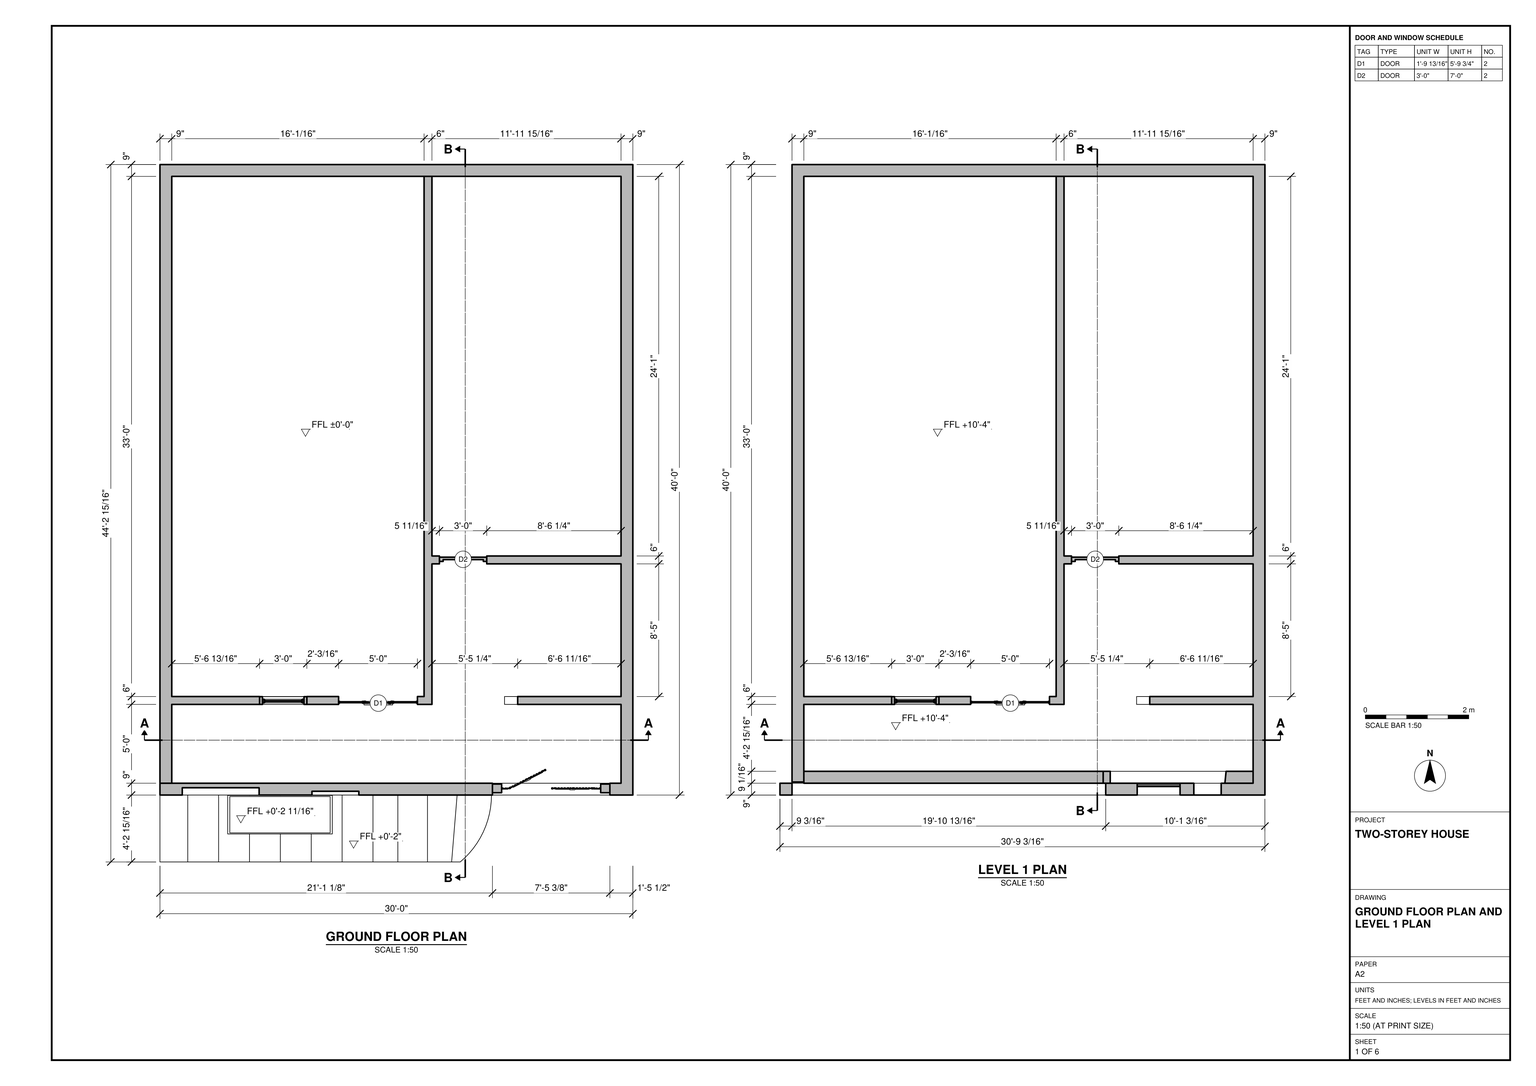
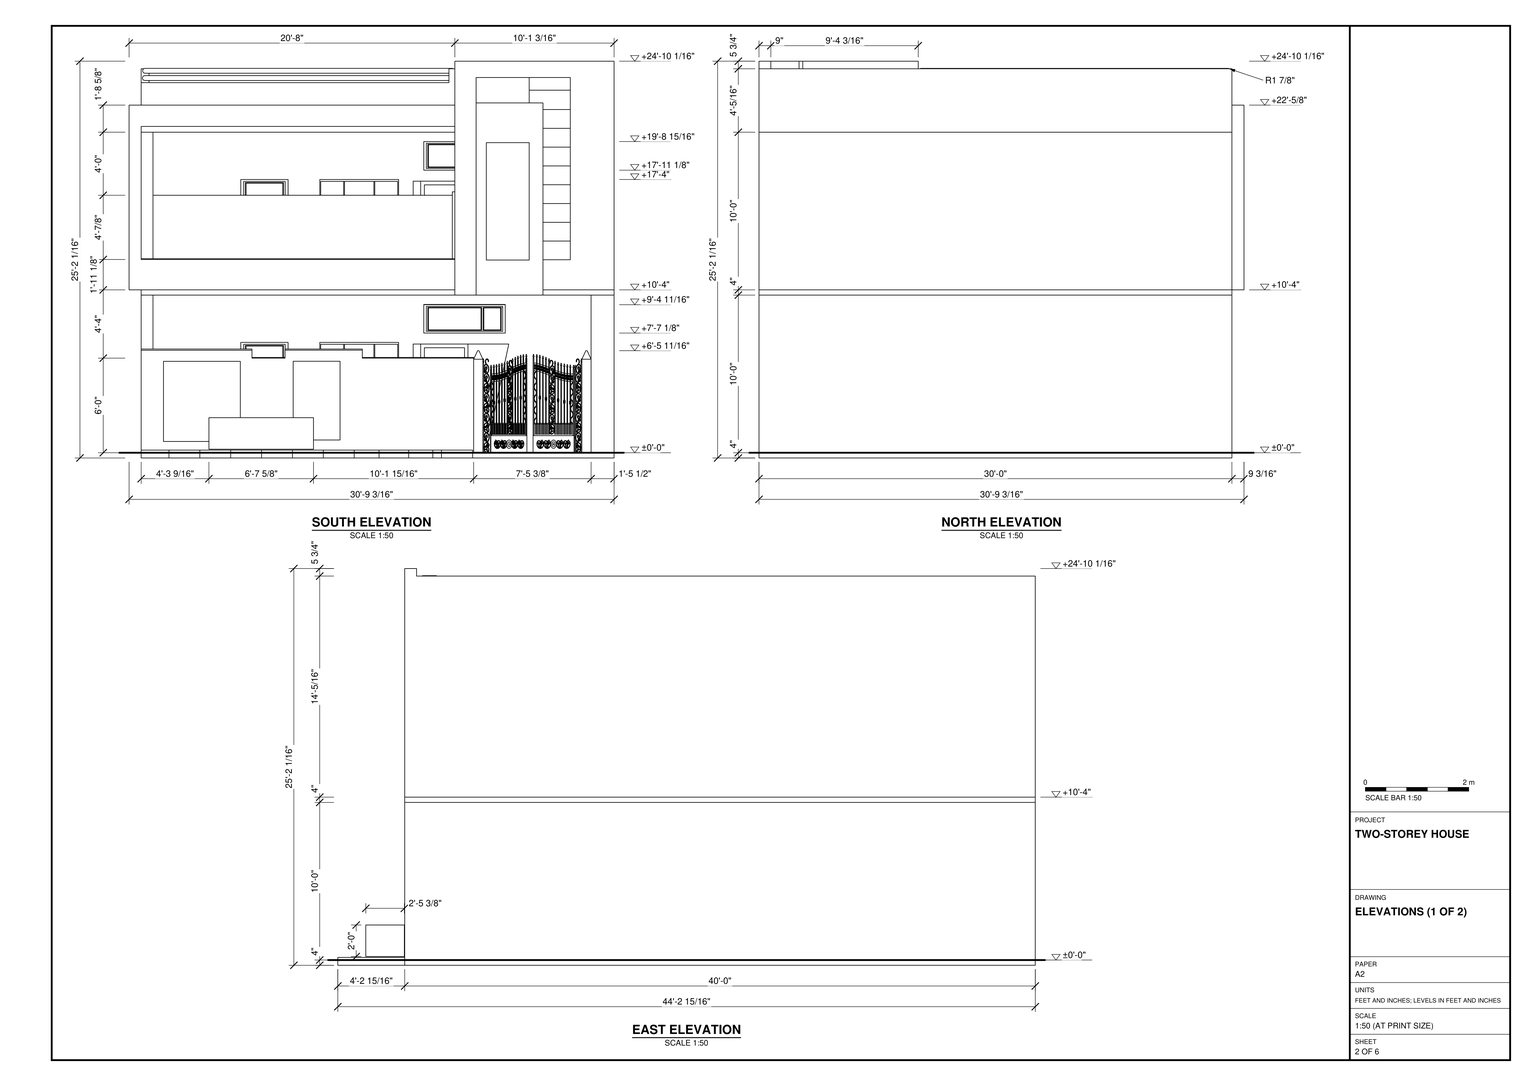
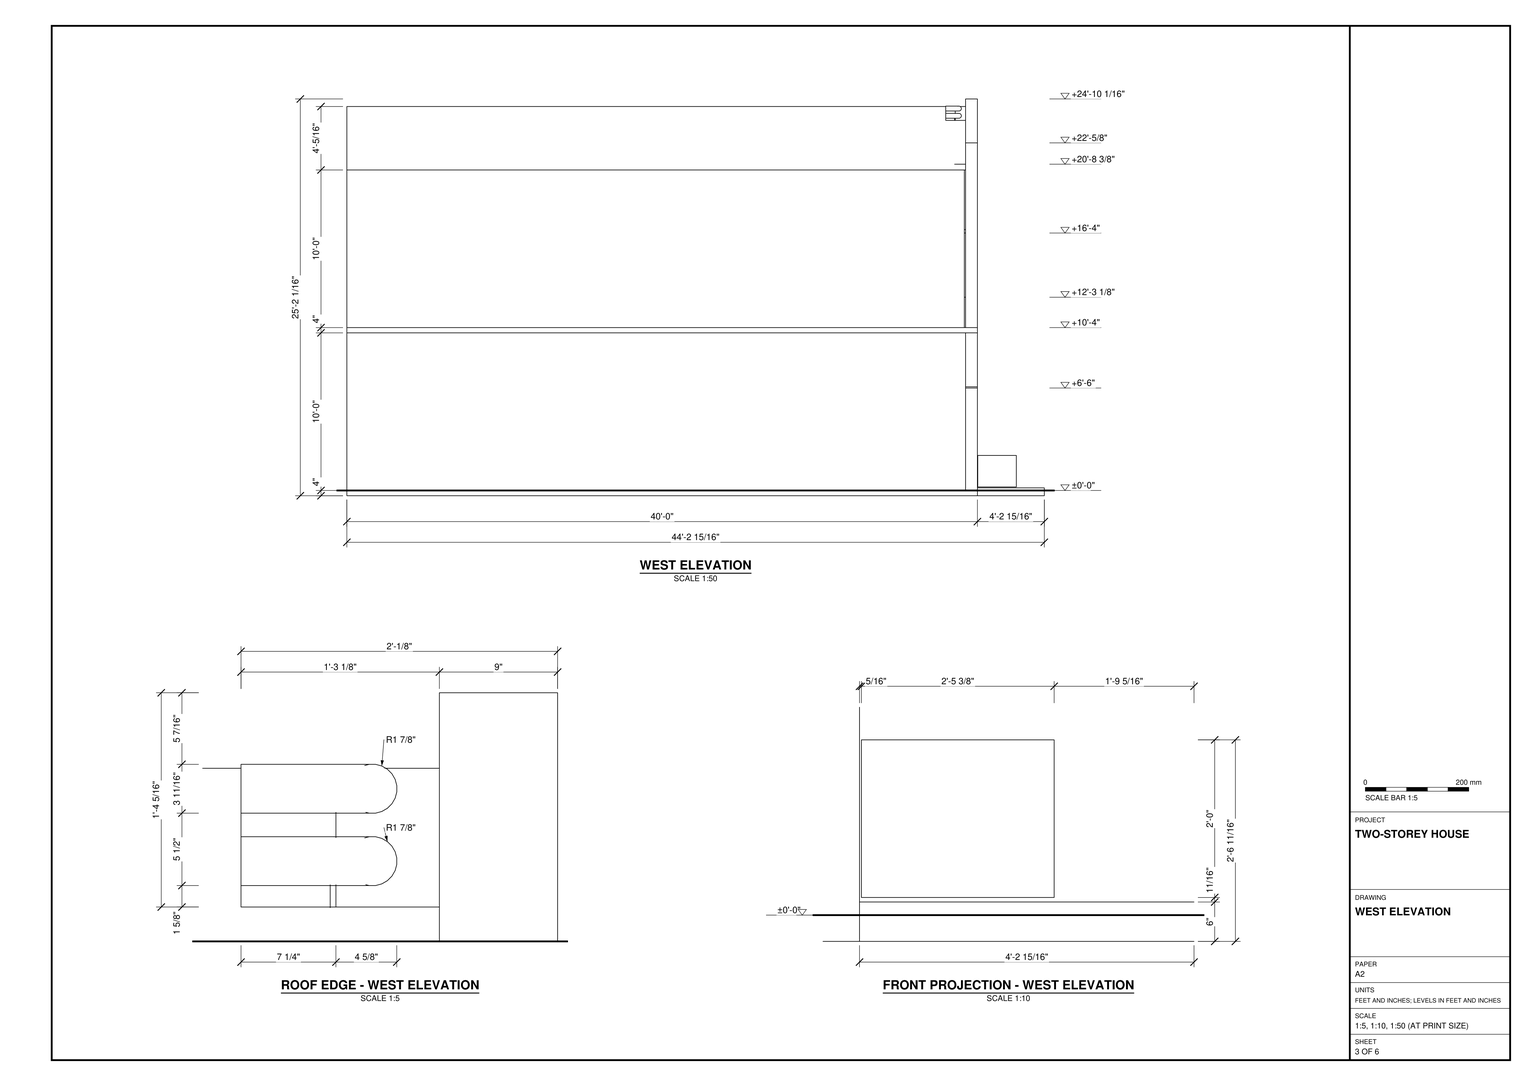
Build the two-storey house in SketchUp using task_files/diagram_01.pdf. Work in feet and inches. Orient the entrance to the south. The overall model, including the front projection and roof edge, measures 30'-9 3/16" east to west, 44'-2 15/16" north to south and 25'-2 1/16" high. Set the ground finished floor at ±0'-0" and the upper finished floor at +10'-4".

Lay out the 9" exterior walls and 6" internal partitions from the plans. On each floor, keep the large room to the west and divide the narrower eastern bay with a cross wall. Model the floor slabs, doors and windows, using the plans to locate the openings and the elevations to set their heights.

At the south entrance, model the projecting paved strip, low solid front wall and paired gate. Above them, form the recessed balcony with its solid front, surrounding rectangular frame and taller panel over the gate. Follow the roof-edge detail for the horizontal bands and their rounded profile.

Keep walls, slabs, roof and each furniture or joinery piece shown in separate groups or components, and use components for repeated parts. Decor and loose items, where shown, may be any suitable library components. Save one SketchUp model as output_files/two_storey_house_with_a_gated_entrance_and_balcony.skp.

# SketchUp Ruby script. Lengths in inches.
U = 1.inch
M = Sketchup.active_model
def pt(a) = Geom::Point3d.new(a.map { |v| v * U })
def face(e, loops, mat)
  f = e.add_face(loops[0].map { |a| pt(a) })
  loops[1..].each { |l| e.add_face(l.map { |a| pt(a) }).erase! }
  f.material = f.back_material = mat if mat
  f
end
# faces: each face lists its corners as indices into pts; further lists are holes
def faces(e, pts, list, mat = nil) = list.each { |f| face(e, (f[0].is_a?(Array) ? f : [f]).map { |l| l.map { |i| pts[i] } }, mat) }
# xy, xz, yz: faces in a plane at the given z, y or x. An outline is a flat list of corners, or four numbers for a rectangle; further outlines are holes
def ring(l) = l.size == 4 ? [[l[0], l[1]], [l[2], l[1]], [l[2], l[3]], [l[0], l[3]]] : l.each_slice(2).to_a
def flat(e, list, mat, &to3) = list.each { |f| face(e, (f[0].is_a?(Array) ? f : [f]).map { |l| ring(l).map { |u, v| to3.(u, v) } }, mat) }
def xy(e, z, list, mat = nil) = flat(e, list, mat) { |x, y| [x, y, z] }
def xz(e, y, list, mat = nil) = flat(e, list, mat) { |x, z| [x, y, z] }
def yz(e, x, list, mat = nil) = flat(e, list, mat) { |y, z| [x, y, z] }
def lines(e, pts, list) = list.each { |a, b| e.add_line(pt(pts[a]), pt(pts[b])) }
# prism: a flat outline (further loops are holes) pulled along v
def prism(e, loops, v, mat = nil)
  f = face(e, loops, mat); d = Geom::Vector3d.new(v.map { |x| x * U })
  f.pushpull(f.normal.samedirection?(d) ? d.length : -d.length)
end
def box(e, o, s, mat = nil) = prism(e, [[o, [o[0] + s[0], o[1], o[2]], [o[0] + s[0], o[1] + s[1], o[2]], [o[0], o[1] + s[1], o[2]]]], [0, 0, s[2]], mat)
def at(x, y, z, deg = 0) = Geom::Transformation.translation(pt([x, y, z])) * Geom::Transformation.rotation(ORIGIN, Z_AXIS, deg.degrees)
def axes(o, x, y, z) = Geom::Transformation.new([*x, 0, *y, 0, *z, 0, *pt(o).to_a, 1])
def part(name) = M.definitions.add(name)
# library, detail: a bought-in or finely detailed component or shape, given as its bounding box
def library(name, o, s) = part(name).tap { |d| box(d.entities, o, s) }
def detail(e, o, s) = box(e.add_group.entities, o, s)
def put(e, d, t, mat = nil) = e.add_instance(d, t).tap { |i| i.material = mat if mat }
def group(e, t, mat = nil) = e.add_group.tap { |g| g.transformation = t; g.material = mat if mat }.entities
root = M.entities
M.materials.add("Portão1").color = [45, 31, 24]
M.materials.add("[Color A01]").color = [255, 204, 204]
M.materials.add("[Color C07]").color = [130, 64, 0]
M.materials.add("[Color D07]").color = [153, 114, 0]
M.materials.add("[Color H01]").color = [204, 255, 255]
M.materials.add("[Color H07]").color = [0, 153, 153]
M.materials.add("[Color M00]").color = [255, 255, 255]
M.materials.add("[Color M05]").color = [114, 114, 114]
M.materials.add("[Color M06]").color = [86, 86, 86]
M.materials.add("[Color M08]").color = [30, 30, 30]
M.materials.add("[Diamond Box]").color = [152, 152, 152]
M.materials.add("[Formica Graystone]").color = [149, 146, 135]
M.materials.add("[Formica Speckled Grey]").color = [94, 105, 111]
M.materials.add("[Metal Corrugated Shiny]").color = [193, 193, 193]
M.materials.add("[Metal Embossed]").color = [144, 144, 144]
M.materials.add("[Metal Seamed]").color = [118, 119, 115]
M.materials.add("[Translucent Glass Blue]").color = [100, 149, 237]
M.materials["[Translucent Glass Blue]"].alpha = 0.5
c1 = library("Framed window",[0,0,0],[45.28,5.91,88.58])
c2 = part("puerta")
xy(c2.entities,0,[[122.07,0.28,122.07,2.03,141.26,2.03,141.26,0.28,139.87,0.28,139.87,1.03,123.57,1.03,123.57,0.28]])
xy(c2.entities,34.05,[[123.57,0.28,139.87,1.03]])
xy(c2.entities,35.79,[[122.07,0.28,141.26,2.03]])
xz(c2.entities,0.28,[[122.07,0,123.57,0,123.57,34.05,139.87,34.05,139.87,0,141.26,0,141.26,35.79,122.07,35.79]])
xz(c2.entities,1.03,[[123.57,0,139.87,34.05]])
xz(c2.entities,2.03,[[122.07,0,141.26,35.79]])
yz(c2.entities,122.07,[[0.28,0,2.03,35.79]])
yz(c2.entities,123.57,[[0.28,0,1.03,34.05]])
yz(c2.entities,139.87,[[0.28,0,1.03,34.05]])
yz(c2.entities,141.26,[[0.28,0,2.03,35.79]])
c3 = part("puerta medieval")
put(c3.entities,c2,axes([-167.24,-2.78,0],[2.37,0,0],[0,2.37,0],[0,0,2.37]))
c4 = library("Group\#4",[0,0,0],[50.79,2.36,34.25])
c5 = library("Group\#50",[0,0,0],[18.9,34.65,18.9])
c6 = library("Group\#125",[0,0,0],[24.7,44.27,7.48])
c7 = part("Group\#121")
xy(c7.entities,0,[[0,0,3.91,91.27]])
xy(c7.entities,3.9375,[[0,0,3.91,91.27]])
yz(c7.entities,0,[[0,0,91.27,3.9375]])
yz(c7.entities,3.91,[[0,0,91.27,3.9375]])
c8 = library("Group\#127",[0,0,0],[67.6,135.77,7.48])
c9 = library("Group\#123",[-2.125,-9.89,0],[28.4375,40.22,7.48])
c10 = library("Group\#134",[0.71,0,0],[33.82,463.5,7.48])
c11 = library("Group\#128",[0,0,0],[67.6,87.29,7.48])
c12 = library("Group\#126",[0,0,0],[79.08,92.15,7.48])
c13 = library("Group\#63",[0,0,0],[9.61,9.61,1.97])
c14 = part("Group\#139")
xy(c14.entities,0,[[0,0,15.75,15.75]])
xy(c14.entities,107.61,[[0,0,15.75,15.75]])
xy(c14.entities,117.46,[[6.69,6.69,9.06,9.06]])
xz(c14.entities,0,[[0,0,15.75,107.61]])
xz(c14.entities,15.75,[[0,0,15.75,107.61]])
yz(c14.entities,0,[[0,0,15.75,107.61]])
yz(c14.entities,15.75,[[0,0,15.75,107.61]])
p = [[15.75,0,107.61],[9.06,6.69,117.46],[6.69,6.69,117.46],[0,0,107.61],[6.69,9.06,117.46],[0,15.75,107.61],
  [15.75,15.75,107.61],[9.06,9.06,117.46]]
faces(c14.entities,p,[[0,1,2,3],[2,4,5,3],[1,0,6,7],[5,4,7,6]])
c15 = library("Group\#133",[0,65.85,0],[33.82,371.91,7.48])
c16 = library("Group\#103",[0,-22.71,0],[10.28,108.02,0.97])
c17 = part("Group\#135")
box(c17.entities,[0,-207.47,0],[11.8125,797.23,11.8125])
c18 = library("Group\#130",[0,0,0],[71.84,113.4,4.25])
c19 = part("Group\#146")
xy(c19.entities,0,[[1.62,1.62,1.62,11.86,2.11,11.86,2.11,2.11],[1.62,1.62,2.11,2.11,235.86,2.11,235.86,1.62]],"[Formica Speckled Grey]")
xy(c19.entities,3.72,[[1.61,1.61,2.1,2.1,2.1,11.86,1.61,11.86],[1.61,1.61,235.86,1.61,235.86,2.1,2.1,2.1]],"[Formica Speckled Grey]")
xz(c19.entities,0,[[0,1.61,235.86,2.1]],"[Formica Speckled Grey]")
xz(c19.entities,3.72,[[3.72,1.62,235.86,2.11]],"[Formica Speckled Grey]")
xz(c19.entities,11.86,[[1.62,0,1.14,0.125,0.72,0.37,0.37,0.72,0.13,1.14,0,1.61,0,2.1,0.125,2.58,0.37,3,0.72,3.35,1.14,3.59,1.61,3.72,2.1,3.72,2.58,3.59,3,3.35,3.35,3,3.59,2.58,3.72,2.11,3.72,1.62,3.59,1.14,3.35,0.72,3,0.37,2.58,0.13,2.11,0]],"[Formica Speckled Grey]")
yz(c19.entities,0,[[0,1.61,11.86,2.1]],"[Formica Speckled Grey]")
yz(c19.entities,3.72,[[3.72,1.62,11.86,2.11]],"[Formica Speckled Grey]")
yz(c19.entities,235.86,[[1.62,0,2.11,0,2.58,0.13,3,0.37,3.35,0.72,3.59,1.14,3.72,1.62,3.72,2.11,3.59,2.58,3.35,3,3,3.35,2.58,3.59,2.1,3.72,1.61,3.72,1.14,3.59,0.72,3.35,0.37,3,0.125,2.58,0,2.1,0,1.61,0.13,1.14,0.37,0.72,0.72,0.37,1.14,0.125]],"[Formica Speckled Grey]")
p = [[1.14,11.86,0.125],[1.62,11.86,0],[1.62,1.62,0],[1.14,1.14,0.125],[235.86,1.62,0],[235.86,1.14,0.125],
  [2.11,11.86,0],[2.58,11.86,0.13],[2.58,2.58,0.13],[2.11,2.11,0],[235.86,2.58,0.13],[235.86,2.11,0],
  [0.72,11.86,0.37],[0.72,0.72,0.37],[235.86,0.72,0.37],[3,11.86,0.37],[3,3,0.37],[235.86,3,0.37],
  [0.37,11.86,0.72],[0.37,0.37,0.72],[235.86,0.37,0.72],[3.35,11.86,0.72],[3.35,3.35,0.72],[235.86,3.35,0.72],
  [0.13,11.86,1.14],[0.13,0.13,1.14],[235.86,0.13,1.14],[3.59,11.86,1.14],[3.59,3.59,1.14],[235.86,3.59,1.14],
  [0,11.86,1.61],[0,0,1.61],[235.86,0,1.61],[3.72,11.86,1.62],[3.72,3.72,1.62],[235.86,3.72,1.62],
  [0.125,11.86,2.58],[0,11.86,2.1],[0,0,2.1],[0.125,0.125,2.58],[235.86,0,2.1],[235.86,0.125,2.58],
  [3.72,11.86,2.11],[3.59,11.86,2.58],[3.59,3.59,2.58],[3.72,3.72,2.11],[235.86,3.59,2.58],[235.86,3.72,2.11],
  [0.37,11.86,3],[0.37,0.37,3],[235.86,0.37,3],[3.35,11.86,3],[3.35,3.35,3],[235.86,3.35,3],
  [0.72,11.86,3.35],[0.72,0.72,3.35],[235.86,0.72,3.35],[3,11.86,3.35],[3,3,3.35],[235.86,3,3.35],
  [1.14,11.86,3.59],[1.14,1.14,3.59],[235.86,1.14,3.59],[2.58,11.86,3.59],[2.58,2.58,3.59],[235.86,2.58,3.59],
  [1.61,11.86,3.72],[1.61,1.61,3.72],[235.86,1.61,3.72],[2.1,11.86,3.72],[2.1,2.1,3.72],[235.86,2.1,3.72]]
faces(c19.entities,p,[[0,1,2,3],[3,2,4,5],[6,7,8,9],[9,8,10,11],[12,0,3,13],[13,3,5,14],[7,15,16,8],[8,16,17,10],
  [18,12,13,19],[19,13,14,20],[15,21,22,16],[16,22,23,17],[24,18,19,25],[25,19,20,26],[21,27,28,22],[22,28,29,23],
  [30,24,25,31],[31,25,26,32],[27,33,34,28],[28,34,35,29],[36,37,38,39],[39,38,40,41],[42,43,44,45],[45,44,46,47],
  [48,36,39,49],[49,39,41,50],[43,51,52,44],[44,52,53,46],[54,48,49,55],[55,49,50,56],[51,57,58,52],[52,58,59,53],
  [60,54,55,61],[61,55,56,62],[57,63,64,58],[58,64,65,59],[66,60,61,67],[67,61,62,68],[63,69,70,64],[64,70,71,65]],"[Formica Speckled Grey]")
xy(root,-4,[[9.1875,0,9.1875,50.9375,261.5625,50.9375,261.38,46.11,260.85,41.3,259.97,36.54,258.75,31.87,257.19,27.29,255.31,22.84,253.1,18.53,250.59,14.4,247.79,10.46,244.71,6.73,241.36,3.24,237.77,0],[9.1875,50.9375,369.1875,530.9375]])
xy(root,0,[[351.7,50.9375,351.7,59.9375,360.1875,59.9375,360.1875,119.9375,271.49,119.9375,271.49,125.9375,360.1875,125.9375,360.1875,226.9375,257.96,226.9375,257.96,232.9375,360.1875,232.9375,360.1875,521.9375,18.1875,521.9375,18.1875,125.9375,121.03,125.9375,121.03,119.9375,18.1875,119.9375,18.1875,59.9375,9.1875,59.9375,9.1875,530.9375,369.1875,530.9375,369.1875,50.9375],[9.1875,50.9375,262.3,59.9375],[121.03,119.9375,145.18,125.9375],[205.18,119.9375,205.18,125.9375,210.25,125.9375,210.25,521.9375,216.25,521.9375,216.25,232.9375,221.96,232.9375,221.96,226.9375,216.25,226.9375,216.25,119.9375]])
xy(root,0,[[18.1875,59.9375,360.1875,59.9375,360.1875,119.9375,271.49,119.9375,271.49,125.9375,360.1875,125.9375,360.1875,226.9375,257.96,226.9375,257.96,232.9375,360.1875,232.9375,360.1875,521.9375,216.25,521.9375,216.25,232.9375,221.96,232.9375,221.96,226.9375,216.25,226.9375,216.25,119.9375,205.18,119.9375,205.18,125.9375,210.25,125.9375,210.25,521.9375,18.1875,521.9375,18.1875,125.9375,145.18,125.9375,145.18,119.9375,18.1875,119.9375]],"[Formica Graystone]")
xy(root,2,[[30.35,0,53.85,50.9375]])
xy(root,2,[[77.35,0,100.85,50.9375],[124.35,0,147.85,50.9375],[171.35,0,190.29,50.9375],[212.84,0,231.21,0,235.39,50.9375,212.84,50.9375]],"[Color M00]")
xy(root,2,[[9.1875,0,30.35,50.9375],[53.85,0,77.35,50.9375],[100.85,0,124.35,50.9375],[147.85,0,171.35,50.9375],[190.29,0,212.84,50.9375],
  [231.21,0,237.77,0,241.36,3.24,244.71,6.73,247.79,10.46,250.59,14.4,253.1,18.53,255.31,22.84,257.19,27.29,258.75,31.87,259.97,36.54,260.85,41.3,261.38,46.11,261.5625,50.9375,235.39,50.9375]],"[Color M08]")
xy(root,8.57,[[26.18,50.9375,84.68,56.5]],"[Color H01]")
xy(root,9.69,[[124.91,50.9375,160.6,53.8125]],"[Color H01]")
xy(root,36,[[85.03,119.9375,121.03,125.9375]])
xy(root,69.57,[[26.18,50.9375,84.68,56.5]],"[Color H01]")
xy(root,69.63,[[124.91,50.9375,160.6,53.8125]],"[Color H01]")
xy(root,72,[[93.55,50.9375,118.71,59.9375],[177.54,50.9375,262.3,59.9375]])
xy(root,72.5625,[[93.55,50.9375,118.71,59.9375],[177.54,50.9375,262.3,59.9375]],"[Color M06]")
xy(root,78,[[9.1875,50.9375,93.55,59.9375]])
xy(root,78.0625,[[118.71,50.9375,177.54,59.9375]])
xy(root,78.9375,[[9.1875,50.9375,93.55,59.9375],[118.71,50.9375,177.54,59.9375]],"[Color M06]")
xy(root,82.74,[[216.25,119.9375,289.02,125.9375]])
xy(root,84,[[85.03,119.9375,121.03,125.9375],[145.18,119.9375,205.18,125.9375],[221.96,226.9375,257.96,232.9375]])
xy(root,91.09,[[224.34,119.9375,286.34,125.9375]])
xy(root,112.91,[[224.34,119.9375,286.34,125.9375]])
xy(root,120,[[9.1875,50.9375,9.1875,59.9375,18.1875,59.9375,18.1875,119.9375,360.1875,119.9375,360.1875,59.9375,351.7,59.9375,351.7,50.9375],[[351.7,50.9375,351.7,59.9375,360.1875,59.9375,360.1875,119.9375,18.1875,119.9375,18.1875,59.9375,9.1875,59.9375,9.1875,530.9375,369.1875,530.9375,369.1875,50.9375],[18.1875,125.9375,210.25,125.9375,210.25,521.9375,216.25,521.9375,216.25,232.9375,360.1875,232.9375,360.1875,521.9375,18.1875,521.9375],[216.25,125.9375,360.1875,226.9375]]],"[Color A01]")
xy(root,124,[[9.1875,59.9375,18.1875,60.875]])
xy(root,124,[[338.55,50.9375,338.55,59.9375,360.1875,59.9375,360.1875,119.9375,271.49,119.9375,271.49,125.9375,360.1875,125.9375,360.1875,226.9375,257.96,226.9375,257.96,232.9375,360.1875,232.9375,360.1875,521.9375,18.1875,521.9375,18.1875,125.9375,121.03,125.9375,121.03,119.9375,18.1875,119.9375,18.1875,60.875,9.1875,60.875,9.1875,530.9375,369.1875,530.9375,369.1875,50.9375],[315.07,50.9375,338.55,59.9375],[121.03,119.9375,145.18,125.9375],[205.18,119.9375,205.18,125.9375,210.25,125.9375,210.25,521.9375,216.25,521.9375,216.25,232.9375,221.96,232.9375,221.96,226.9375,216.25,226.9375,216.25,119.9375]],"[Color A01]")
xy(root,124,[[0,50.9375,9.1875,59.9375]],"[Color M06]")
xy(root,124,[[18.1875,59.9375,152.7,69],[152.7,59.9375,246.05,69],[246.05,59.9375,251.43,69],[251.43,59.9375,338.7,59.9375,339.625,69,251.43,69],[18.1875,69,360.1875,69,360.1875,119.9375,271.49,119.9375,271.49,125.9375,360.1875,125.9375,360.1875,226.9375,257.96,226.9375,257.96,232.9375,360.1875,232.9375,360.1875,521.9375,216.25,521.9375,216.25,232.9375,221.96,232.9375,221.96,226.9375,216.25,226.9375,216.25,119.9375,205.18,119.9375,205.18,125.9375,210.25,125.9375,210.25,521.9375,18.1875,521.9375,18.1875,125.9375,145.18,125.9375,145.18,119.9375,18.1875,119.9375]],"[Formica Graystone]")
xy(root,146.7,[[271.96,50.9375,304.58,57.4375]],"[Color M00]")
xy(root,146.7,[[271.96,57.4375,304.58,57.6875],[271.96,57.6875,304.58,59.4375]],"[Color M06]")
xy(root,146.92,[[315.07,50.9375,335.88,59.9375]],"[Color A01]")
xy(root,147.125,[[9.1875,50.9375,247.99,59.9375]],"[Color M06]")
xy(root,147.6875,[[9.1875,50.9375,247.99,59.9375]],"[Color H07]")
xy(root,160,[[85.03,119.9375,121.03,125.9375]],"[Color A01]")
xy(root,196,[[338.7,59.9375,360.1875,59.9375,360.1875,69,339.625,69]],"[Formica Graystone]")
xy(root,196,[[18.1875,59.9375,246.05,69]],"[Metal Seamed]")
xy(root,198.625,[[246.05,59.9375,251.43,69]],"[Metal Seamed]")
xy(root,206.74,[[216.25,119.9375,289.02,125.9375]],"[Color H01]")
xy(root,208,[[85.03,119.9375,121.03,125.9375],[145.18,119.9375,205.18,125.9375],[221.96,226.9375,257.96,232.9375]],"[Color A01]")
xy(root,215.09,[[224.34,119.9375,286.34,125.9375]],"[Color A01]")
xy(root,236.07,[[271.96,50.9375,304.58,57.4375]],"[Color M00]")
xy(root,236.07,[[271.96,57.4375,304.58,57.6875],[271.96,57.6875,304.58,59.4375]],"[Color M06]")
xy(root,236.91,[[224.34,119.9375,286.34,125.9375]],"[Color A01]")
xy(root,244,[[9.1875,59.9375,9.1875,60.875,18.1875,60.875,18.1875,119.9375,360.1875,119.9375,360.1875,59.9375,335.88,59.9375,335.88,68.25,315.07,68.25,315.07,59.9375]])
xy(root,248.4,[[9.1875,50.9375,247.99,59.9375]],"[Color A01]")
xy(root,264.625,[[0,50.9375,247.99,59.9375]],"[Color M06]")
xy(root,266.3125,[[264.16,59.9375,315.07,68.25]],"[Color A01]")
xy(root,266.3125,[[264.16,50.9375,315.07,59.9375]],"[Color M05]")
xy(root,275.75,[[15.1875,67.8125,363.1875,524.9375]],"[Formica Speckled Grey]")
xy(root,281.75,[[9.1875,59.9375,243.47,59.9375,243.47,67.8125,15.1875,67.8125,15.1875,75.04,9.1875,75.04]],"[Color H01]")
xy(root,285.66,[[264.16,50.9375,335.88,59.9375],[264.16,59.9375,335.88,68.25]],"[Color A01]")
xy(root,292.3125,[[243.47,59.9375,369.1875,59.9375,369.1875,530.9375,9.1875,530.9375,9.1875,75.04,15.1875,75.04,15.1875,524.9375,363.1875,524.9375,363.1875,67.8125,243.47,67.8125]],"[Color H01]")
xy(root,298.0625,[[247.99,50.9375,369.1875,59.9375]],"[Color H01]")
xz(root,0,[[30.35,-4,53.85,2],[77.35,-4,100.85,2],[124.35,-4,147.85,2],[171.35,-4,190.29,2],[212.84,-4,231.21,2]])
xz(root,0,[[9.1875,-4,30.35,2],[53.85,-4,77.35,2],[100.85,-4,124.35,2],[147.85,-4,171.35,2],[190.29,-4,212.84,2],
  [231.21,-4,237.77,2]],"[Color M08]")
xz(root,50.9375,[[9.1875,-4,261.5625,0],[9.1875,0,261.5625,2]])
xz(root,50.9375,[[9.1875,147.125,247.99,147.6875]],"[Color A01]")
xz(root,50.9375,[[315.07,146.92,335.88,161.15],[315.07,161.15,335.88,175.4],[315.07,175.4,335.88,189.71],[315.07,189.71,335.88,204.03],[315.07,204.03,335.88,218.34],
  [315.07,218.34,335.88,232.65],[315.07,232.65,335.88,246.96],[315.07,246.96,335.88,261.28],[315.07,261.28,335.88,261.28,335.88,275.99,304.58,275.99,304.58,266.3125,315.07,266.3125],[304.58,275.99,335.88,285.66]],"[Color C07]")
xz(root,50.9375,[[9.1875,120,247.99,124]],"[Color D07]")
xz(root,50.9375,[[261.5625,-4,369.1875,0],[351.7,0,369.1875,120],[315.07,120,369.1875,124]],"[Color H01]")
xz(root,50.9375,[[[261.5625,0,262.3,0,262.3,72,177.54,72,177.54,78.0625,118.71,78.0625,118.71,72,93.55,72,93.55,78,9.1875,78,9.1875,2,261.5625,2],[26.18,8.57,84.68,69.57],[124.91,9.69,160.6,69.63]],[247.99,120,264.16,120,264.16,285.66,335.88,285.66,335.88,146.92,315.07,146.92,315.07,124,369.1875,124,369.1875,298.0625,247.99,298.0625]],"[Color H07]")
xz(root,50.9375,[[93.55,72,118.71,72.5625],[177.54,72,262.3,72.5625],[9.1875,78,93.55,78.9375],[118.71,78.0625,177.54,78.9375],[[264.16,120,315.07,266.3125],[271.96,146.7,304.58,236.07]],
  [0,124,247.99,124,247.99,147.125,9.1875,147.125,9.1875,248.4,247.99,248.4,247.99,264.625,0,264.625]],"[Color M06]")
xz(root,50.9375,[[264.16,266.3125,304.58,285.66]],"[Diamond Box]")
xz(root,53.8125,[[124.91,9.69,160.6,69.63]],"[Color H01]")
xz(root,56.5,[[26.18,8.57,84.68,69.57]],"[Color H01]")
xz(root,57.4375,[[271.96,146.7,304.58,236.07]],"[Color A01]")
xz(root,57.6875,[[271.96,146.7,304.58,236.07]],"[Color M06]")
xz(root,59.4375,[[271.96,146.7,304.58,236.07]],"[Color M06]")
xz(root,59.9375,[[9.1875,0,18.1875,78],[18.1875,0,18.1875,78,93.55,78,93.55,72,118.71,72,118.71,78.0625,177.54,78.0625,177.54,72,262.3,72,262.3,0],[351.7,0,360.1875,120],[93.55,72,118.71,72.5625],[177.54,72,262.3,72.5625],
  [9.1875,78,18.1875,78.9375]])
xz(root,59.9375,[[0,124,18.1875,124,18.1875,147.125,9.1875,147.125,9.1875,264.625,0,264.625],[152.7,124,246.05,147.125],[246.05,124,247.99,147.125],[251.43,124,251.43,198.625,247.99,198.625,247.99,244,264.16,244,264.16,124],[315.07,124,315.07,146.92,335.88,146.92,335.88,196,338.7,196,338.7,124],
  [18.1875,147.6875,246.05,196],[335.88,196,360.1875,244],[247.99,244,247.99,292.3125,335.88,292.3125,335.88,285.66,264.16,285.66,264.16,244],[264.16,244,315.07,266.3125],[335.88,244,338.7,292.3125],
  [338.7,244,360.1875,292.3125],[9.1875,248.4,247.99,250],[9.1875,250,247.99,264.625],[335.88,292.3125,338.7,298.0625],[338.7,292.3125,360.1875,298.0625],
  [360.1875,292.3125,369.1875,298.0625]],"[Color A01]")
xz(root,59.9375,[[9.1875,78.9375,18.1875,120]],"[Color H01]")
xz(root,59.9375,[[9.1875,244,247.99,248.4],[9.1875,264.625,247.99,264.625,247.99,292.3125,243.47,292.3125,243.47,281.75,9.1875,281.75]],"[Color H07]")
xz(root,59.9375,[[264.16,124,315.07,244]],"[Color M05]")
xz(root,59.9375,[[18.1875,78,93.55,78.9375],[118.71,78.0625,177.54,78.9375],[9.1875,147.125,18.1875,147.6875],[18.1875,147.125,152.7,147.6875],[152.7,147.125,246.05,147.6875],
  [246.05,147.125,247.99,147.6875]],"[Color M06]")
xz(root,59.9375,[[18.1875,124,152.7,147.125],[247.99,124,251.43,198.625],[338.7,124,360.1875,196]],"[Formica Graystone]")
xz(root,59.9375,[[247.99,292.3125,335.88,298.0625]],"[Formica Speckled Grey]")
xz(root,59.9375,[[246.05,147.6875,247.99,198.625]],"[Metal Seamed]")
xz(root,60.875,[[9.1875,124,18.1875,244]],"[Color H07]")
xz(root,67.8125,[[15.1875,275.75,15.1875,281.75,243.47,281.75,243.47,292.3125,363.1875,292.3125,363.1875,275.75]],"[Color H01]")
xz(root,68.25,[[315.07,244,335.88,244,335.88,285.66,264.16,285.66,264.16,266.3125,315.07,266.3125]],"[Color A01]")
xz(root,69,[[339.625,124,360.1875,196]],"[Formica Graystone]")
xz(root,69,[[246.05,124,251.43,198.625]],"[Metal Seamed]")
xz(root,69,[[18.1875,124,246.05,196]],"[Translucent Glass Blue]")
xz(root,75.04,[[9.1875,281.75,15.1875,292.3125]],"[Color H01]")
xz(root,119.9375,[[[18.1875,0,145.18,0,145.18,84,205.18,84,205.18,0,216.25,0,216.25,82.74,289.02,82.74,271.49,0,360.1875,0,360.1875,120,18.1875,120],[85.03,36,121.03,84],[224.34,91.09,286.34,112.91]],[[18.1875,124,145.18,124,145.18,208,205.18,208,205.18,124,216.25,124,216.25,206.74,289.02,206.74,271.49,124,360.1875,124,360.1875,244,18.1875,244],[85.03,160,121.03,208],[224.34,215.09,286.34,236.91]]],"[Color H01]")
xz(root,125.9375,[[[18.1875,0,18.1875,120,210.25,120,210.25,0,205.18,0,205.18,84,145.18,84,145.18,0],[85.03,36,121.03,84]],[[271.49,0,289.02,82.74,216.25,82.74,216.25,120,360.1875,120,360.1875,0],[224.34,91.09,286.34,112.91]],[[18.1875,124,18.1875,244,210.25,244,210.25,124,205.18,124,205.18,208,145.18,208,145.18,124],[85.03,160,121.03,208]],[[271.49,124,289.02,206.74,216.25,206.74,216.25,244,360.1875,244,360.1875,124],[224.34,215.09,286.34,236.91]]],"[Color A01]")
xz(root,226.9375,[[216.25,0,221.96,0,221.96,84,257.96,84,257.96,0,360.1875,0,360.1875,120,216.25,120],[216.25,124,221.96,124,221.96,208,257.96,208,257.96,124,360.1875,124,360.1875,244,216.25,244]],"[Color H01]")
xz(root,232.9375,[[216.25,0,216.25,120,360.1875,120,360.1875,0,257.96,0,257.96,84,221.96,84,221.96,0],[216.25,124,216.25,244,360.1875,244,360.1875,124,257.96,124,257.96,208,221.96,208,221.96,124]],"[Color A01]")
xz(root,521.9375,[[210.25,0,216.25,120]])
xz(root,521.9375,[[18.1875,0,210.25,120],[216.25,0,360.1875,120],[18.1875,124,210.25,244],[210.25,124,216.25,244],[216.25,124,360.1875,244]],"[Color A01]")
xz(root,524.9375,[[15.1875,275.75,363.1875,292.3125]],"[Color H01]")
xz(root,530.9375,[[9.1875,-4,369.1875,0]])
xz(root,530.9375,[[9.1875,0,369.1875,120],[9.1875,120,369.1875,124],[9.1875,124,369.1875,244],[9.1875,244,369.1875,292.3125]],"[Color M00]")
yz(root,0,[[50.9375,124,59.9375,264.625]],"[Color M06]")
yz(root,9.1875,[[0,-4,50.9375,2],[50.9375,0,59.9375,78]])
yz(root,9.1875,[[50.9375,-4,530.9375,0],[59.9375,0,530.9375,120],[50.9375,120,530.9375,124],[60.875,124,530.9375,244],[59.9375,244,59.9375,281.75,75.04,281.75,75.04,292.3125,530.9375,292.3125,530.9375,244]],"[Color M00]")
yz(root,9.1875,[[50.9375,78,59.9375,78.9375],[50.9375,147.125,59.9375,147.6875],[50.9375,147.6875,59.9375,248.4]],"[Color M06]")
yz(root,15.1875,[[67.8125,275.75,524.9375,275.75,524.9375,292.3125,75.04,292.3125,75.04,281.75,67.8125,281.75]],"[Color H01]")
yz(root,18.1875,[[59.9375,0,119.9375,120]])
yz(root,18.1875,[[125.9375,0,521.9375,120],[125.9375,124,521.9375,244]],"[Color A01]")
yz(root,18.1875,[[69,124,119.9375,124,119.9375,244,60.875,244,60.875,196,69,196]],"[Color H01]")
yz(root,18.1875,[[59.9375,124,60.875,196],[60.875,124,69,196]],"[Formica Graystone]")
yz(root,26.18,[[50.9375,8.57,56.5,69.57]],"[Color H01]")
yz(root,84.68,[[50.9375,8.57,56.5,69.57]],"[Color H01]")
yz(root,85.03,[[119.9375,36,125.9375,84]])
yz(root,85.03,[[119.9375,160,125.9375,208]],"[Color A01]")
yz(root,93.55,[[50.9375,72,59.9375,72.5625]])
yz(root,93.55,[[50.9375,72.5625,59.9375,78],[50.9375,78,59.9375,78.9375]],"[Color M06]")
yz(root,118.71,[[50.9375,72,59.9375,72.5625]])
yz(root,118.71,[[50.9375,72.5625,59.9375,78.0625],[50.9375,78.0625,59.9375,78.9375]],"[Color M06]")
yz(root,121.03,[[119.9375,36,125.9375,84]])
yz(root,121.03,[[119.9375,160,125.9375,208]],"[Color A01]")
yz(root,124.91,[[50.9375,9.69,53.8125,69.63]],"[Color H01]")
yz(root,145.18,[[119.9375,0,125.9375,84]])
yz(root,145.18,[[119.9375,124,125.9375,208]],"[Color A01]")
yz(root,160.6,[[50.9375,9.69,53.8125,69.63]],"[Color H01]")
yz(root,177.54,[[50.9375,72,59.9375,72.5625]])
yz(root,177.54,[[50.9375,72.5625,59.9375,78.0625],[50.9375,78.0625,59.9375,78.9375]],"[Color M06]")
yz(root,205.18,[[119.9375,0,125.9375,84]])
yz(root,205.18,[[119.9375,124,125.9375,208]],"[Color A01]")
yz(root,210.25,[[125.9375,0,521.9375,120],[125.9375,124,521.9375,244]],"[Color A01]")
yz(root,216.25,[[232.9375,0,512.5,120],[512.5,0,521.9375,120],[119.9375,124,125.9375,206.74],[125.9375,124,226.9375,244],[232.9375,124,512.5,244],
  [512.5,124,521.9375,244]],"[Color A01]")
yz(root,216.25,[[119.9375,0,125.9375,82.74],[125.9375,0,226.9375,120]],"[Color H01]")
yz(root,221.96,[[226.9375,0,232.9375,84]])
yz(root,221.96,[[226.9375,124,232.9375,208]],"[Color A01]")
yz(root,224.34,[[119.9375,91.09,125.9375,112.91]])
yz(root,224.34,[[119.9375,215.09,125.9375,236.91]],"[Color A01]")
yz(root,243.47,[[59.9375,281.75,67.8125,292.3125]],"[Color H01]")
yz(root,246.05,[[59.9375,124,69,196],[59.9375,196,69,198.625]],"[Formica Graystone]")
yz(root,247.99,[[50.9375,248.4,59.9375,264.625]],"[Color A01]")
yz(root,247.99,[[50.9375,264.625,59.9375,298.0625]],"[Color H01]")
yz(root,247.99,[[50.9375,147.6875,59.9375,248.4]],"[Color H07]")
yz(root,247.99,[[50.9375,147.125,59.9375,147.6875]],"[Color M06]")
yz(root,251.43,[[59.9375,124,69,198.625]],"[Metal Seamed]")
yz(root,257.96,[[226.9375,0,232.9375,84]])
yz(root,257.96,[[226.9375,124,232.9375,208]],"[Color A01]")
yz(root,262.3,[[50.9375,0,59.9375,72],[50.9375,72,59.9375,72.5625]])
yz(root,264.16,[[50.9375,266.3125,59.9375,285.66],[59.9375,266.3125,68.25,285.66]],"[Color A01]")
yz(root,271.96,[[50.9375,146.7,57.4375,236.07]],"[Color M00]")
yz(root,271.96,[[57.4375,146.7,57.6875,236.07],[57.6875,146.7,59.4375,236.07]],"[Color M06]")
yz(root,286.34,[[119.9375,91.09,125.9375,112.91]])
yz(root,286.34,[[119.9375,215.09,125.9375,236.91]],"[Color A01]")
yz(root,304.58,[[50.9375,146.7,57.4375,236.07]],"[Color M00]")
yz(root,304.58,[[57.4375,146.7,57.6875,236.07],[57.6875,146.7,59.4375,236.07]],"[Color M06]")
yz(root,315.07,[[50.9375,124,59.9375,146.92],[59.9375,244,68.25,266.3125]],"[Color A01]")
yz(root,315.07,[[50.9375,146.92,59.9375,266.3125]],"[Color M05]")
yz(root,335.88,[[50.9375,146.92,59.9375,285.66],[59.9375,244,68.25,285.66]],"[Color A01]")
yz(root,351.7,[[50.9375,0,59.9375,120]],"[Color H01]")
yz(root,360.1875,[[125.9375,0,226.9375,120],[232.9375,0,521.9375,120],[69,124,69,196,59.9375,196,59.9375,244,119.9375,244,119.9375,124],[125.9375,124,226.9375,244],[232.9375,124,521.9375,244]],"[Color A01]")
yz(root,360.1875,[[59.9375,0,119.9375,120]],"[Color H01]")
yz(root,360.1875,[[59.9375,124,69,196]],"[Formica Graystone]")
yz(root,363.1875,[[67.8125,275.75,524.9375,292.3125]],"[Color H01]")
yz(root,369.1875,[[50.9375,-4,530.9375,0],[50.9375,0,530.9375,120],[50.9375,120,530.9375,124],[50.9375,124,530.9375,124,530.9375,292.3125,59.9375,292.3125,59.9375,298.0625,50.9375,298.0625]],"[Color M00]")
p = [[237.77,0,-4],[241.36,3.24,-4],[241.36,3.24,2],[237.77,0,2],[244.71,6.73,-4],[244.71,6.73,2],
  [247.79,10.46,-4],[247.79,10.46,2],[250.59,14.4,-4],[250.59,14.4,2],[253.1,18.53,-4],[253.1,18.53,2],
  [255.31,22.84,-4],[255.31,22.84,2],[257.19,27.29,-4],[257.19,27.29,2],[258.75,31.87,-4],[258.75,31.87,2],
  [259.97,36.54,-4],[259.97,36.54,2],[260.85,41.3,-4],[260.85,41.3,2],[261.38,46.11,-4],[261.38,46.11,2],
  [261.5625,50.9375,-4],[261.5625,50.9375,0],[261.5625,50.9375,2],[271.49,119.9375,0],[289.02,119.9375,82.74],[289.02,125.9375,82.74],
  [271.49,125.9375,0],[339.625,69,124],[338.7,59.9375,124],[338.7,59.9375,196],[339.625,69,196],[271.49,119.9375,124],
  [289.02,119.9375,206.74],[289.02,125.9375,206.74],[271.49,125.9375,124],[360.1875,67.54,244],[369.1875,67.54,244],[9.1875,60.875,147.125],
  [9.1875,59.9375,147.125],[247.99,59.9375,124],[247.99,59.9375,121.4375],[9.1875,59.9375,248.4],[9.1875,68.3125,248.4]]
faces(root,p,[[0,1,2,3],[1,4,5,2],[4,6,7,5],[6,8,9,7],[8,10,11,9],[10,12,13,11],[12,14,15,13],[14,16,17,15],
  [16,18,19,17],[18,20,21,19],[20,22,23,21],[22,24,25,26,23]],"[Color M08]")
faces(root,p,[[27,28,29,30],[35,36,37,38]],"[Color H01]")
faces(root,p,[[31,32,33,34]],"[Formica Graystone]")
lines(root,p,[[39,40],[41,42],[43,44],[45,46]])
put(root,c1,axes([286.34,120.49,91.09],[0,0,0.47695],[0,1.47094,0],[-0.69991,0,0]))
put(root,c1,axes([85.03,119.9375,36],[0.79538,0,0],[0,1,0],[0,0,0.54187]))
put(root,c3,axes([125.3125,230.44,0],[0.7917,0,0],[0,0.78,0],[0,0,0.99023]))
put(root,c1,axes([85.03,119.9375,160],[0.79538,0,0],[0,1,0],[0,0,0.54187]),"[Color A01]")
put(root,c1,axes([286.36,120.4,215.09],[0,0,0.48177],[0,1.4858,0],[-0.70009,0,0]),"[Color A01]")
put(root,c3,axes([125.3125,230.44,124],[0.7917,0,0],[0,0.78,0],[0,0,0.99023]),"[Color A01]")
g1 = group(root,at(60.77,21.3,2.6875),"[Color H07]")
xy(g1,0,[[[0,0,79.6,29.35],[1.6,0.84,78,28.51]],[1.6,0.84,78,28.51]])
xy(g1,24,[[[0,0,79.6,29.35],[1.6,0.84,78,28.51]]])
xz(g1,0,[[0,0,79.6,24]])
xz(g1,0.84,[[1.6,0,78,24]])
xz(g1,28.51,[[1.6,0,78,24]])
xz(g1,29.35,[[0,0,79.6,24]])
yz(g1,0,[[0,0,29.35,24]])
yz(g1,1.6,[[0.84,0,28.51,24]])
yz(g1,78,[[0.84,0,28.51,24]])
yz(g1,79.6,[[0,0,29.35,24]])
put(root,c4,axes([145.18,119.56,0],[1.1814,0,0],[0,1.16,0],[0,0,2.45241]),"[Color H01]")
g2 = group(root,at(262.3,52.72,0))
put(g2,c5,axes([46.11,3.81,72.02],[-0.05783,0,0],[0,0,0.08598],[0,-0.05442,0]),"Portão1")
g3 = group(g2,at(75.73,3.62,54.11),"Portão1")
prism(g3,[[[0,-0.64,1.18],[0,-0.64,0],[-1.4375,-0.64,0.04],[-2.88,-0.64,0.15],[-4.3125,-0.64,0.3],[-5.75,-0.64,0.52],[-7.17,-0.64,0.79],[-8.6,-0.64,1.11],[-10.01,-0.64,1.5],[-11.42,-0.64,1.93],[-12.82,-0.64,2.43],[-14.22,-0.64,2.97],[-15.6,-0.64,3.58],[-16.97,-0.64,4.23],[-18.01,-0.64,4.74],[-19.0625,-0.64,5.22],[-20.12,-0.64,5.67],[-21.18,-0.64,6.09],[-22.25,-0.64,6.49],[-23.32,-0.64,6.86],[-24.39,-0.64,7.2],[-25.47,-0.64,7.51],[-26.56,-0.64,7.79],[-27.64,-0.64,8.04],[-28.73,-0.64,8.27],[-29.82,-0.64,8.46],[-29.82,-0.64,9.65],[-29.5,-0.64,9.59],[-28.73,-0.64,9.45],[-27.64,-0.64,9.23],[-26.56,-0.64,8.97],[-25.47,-0.64,8.69],[-24.39,-0.64,8.38],[-23.32,-0.64,8.04],[-22.25,-0.64,7.67],[-21.18,-0.64,7.28],[-20.12,-0.64,6.86],[-19.0625,-0.64,6.4],[-18.01,-0.64,5.92],[-16.97,-0.64,5.42],[-15.6,-0.64,4.76],[-14.22,-0.64,4.16],[-12.82,-0.64,3.61],[-11.42,-0.64,3.12],[-10.01,-0.64,2.68],[-8.6,-0.64,2.3],[-7.17,-0.64,1.97],[-5.75,-0.64,1.7],[-4.3125,-0.64,1.49],[-2.88,-0.64,1.33],[-1.4375,-0.64,1.23]]],[0,0.64,0])
g4 = group(g2,at(45.91,3.62,21.3125),"Portão1")
box(g4,[-0.68,-0.64,-8.29],[0.68,0.64,59])
g5 = group(g2,at(53.28,3.93,20.66),"Portão1")
g6 = group(g5,at(-0.33,-0.3125,0))
box(g6,[-0.43,-0.41,-6.72],[0.43,0.41,56.72])
put(g5,c5,axes([0,0,50],[-0.05783,0,0],[0,0,0.08598],[0,-0.05442,0]))
g7 = group(g2,at(50.91,3.93,21.39),"Portão1")
g8 = group(g7,at(-0.33,-0.3125,0))
box(g8,[-0.43,-0.41,-7.45],[0.43,0.41,57.45])
put(g7,c5,axes([0,0,50],[-0.05783,0,0],[0,0,0.08598],[0,-0.05442,0]))
g9 = group(g2,at(74.1,3.93,13.9375),"Portão1")
g10 = group(g9,at(-0.33,-0.3125,0))
box(g10,[-0.43,-0.41,0],[0.43,0.41,50])
put(g9,c5,axes([0,0,50],[-0.05783,0,0],[0,0,0.08598],[0,-0.05442,0]))
put(g2,c6,axes([55.74,3.62,39.12],[-0.05783,0,0],[0,0,0.08598],[0,-0.05442,0]),"Portão1")
put(g2,c7,axes([70.25,3.62,13.9375],[-0.05783,0,0],[0,0,0.08598],[0,-0.05442,0]),"Portão1")
put(g2,c8,axes([61.61,3.62,58.79],[-0.05783,0,0],[0,0,0.08598],[0,-0.05442,0]),"Portão1")
g11 = group(g2,at(75.42,3.62,55.41),"Portão1")
put(g11,c9,axes([-3.6,0,0.96],[0.05783,0,0],[0,0,0.08598],[0,-0.02721,0]))
put(g11,c9,axes([-8.15,0,1.7],[0.05783,0,0],[0,0,0.08598],[0,-0.02721,0]))
put(g11,c9,axes([-4.67,0,1.29],[-0.05783,0,0],[0,0,0.08598],[0,-0.02721,0]))
put(g11,c9,axes([-12.86,0,3.1],[0.05783,0,0],[0,0,0.08598],[0,-0.02721,0]))
put(g11,c9,axes([-26.78,0,8.54],[0.05783,0,0],[0,0,0.08598],[0,-0.02721,0]))
put(g11,c9,axes([-0.12,0,0.85],[-0.05783,0,0],[0,0,0.08598],[0,-0.02721,0]))
put(g11,c9,axes([-22.13,0,7.09],[0.05783,0,0],[0,0,0.08598],[0,-0.02721,0]))
put(g11,c9,axes([-18.65,0,6.21],[-0.05783,0,0],[0,0,0.08598],[0,-0.02721,0]))
put(g11,c9,axes([-9.39,0,2.39],[-0.05783,0,0],[0,0,0.08598],[0,-0.02721,0]))
put(g11,c9,axes([-23.31,0,7.95],[-0.05783,0,0],[0,0,0.08598],[0,-0.02721,0]))
put(g11,c9,axes([-29.07,-0.01,9.02],[0.05783,0,0],[0,0,0.08598],[0,-0.02721,0]))
g12 = group(g2,at(64.83,3.93,15.875),"Portão1")
g13 = group(g12,at(-0.33,-0.3125,0))
box(g13,[-0.43,-0.41,-1.94],[0.43,0.41,51.94])
put(g12,c5,axes([0,0,50],[-0.05783,0,0],[0,0,0.08598],[0,-0.05442,0]))
put(g2,c10,axes([47.9,3.62,22.44],[-0.05783,0,0],[0,0,0.08598],[0,-0.05442,0]),"Portão1")
put(g2,c11,axes([61.32,3.62,21.73],[-0.05783,0,0],[0,0,0.08598],[0,-0.05442,0]),"Portão1")
put(g2,c12,axes([61.72,3.62,44.16],[-0.05783,0,0],[0,0,0.08598],[0,-0.05442,0]),"Portão1")
put(g2,c11,axes([61.32,3.62,36.75],[-0.05783,0,0],[0,0,0.08598],[0,-0.05442,0]),"Portão1")
put(g2,c12,axes([61.72,3.62,14.04],[-0.05783,0,0],[0,0,0.08598],[0,-0.05442,0]),"Portão1")
put(g2,c11,axes([61.32,3.62,51.85],[-0.05783,0,0],[0,0,0.08598],[0,-0.05442,0]),"Portão1")
put(g2,c12,axes([68.22,2.97,3.17],[0,0,0.08598],[0.05783,0,0],[0,-0.05442,0]),"Portão1")
g14 = group(g2,at(69.55,3.93,14.74),"Portão1")
g15 = group(g14,at(-0.33,-0.3125,0))
box(g15,[-0.43,-0.41,-0.8],[0.43,0.41,50.8])
put(g14,c5,axes([0,0,50],[-0.05783,0,0],[0,0,0.08598],[0,-0.05442,0]))
put(g2,c12,axes([62.93,2.97,3.17],[0,0,0.08598],[0.05783,0,0],[0,-0.05442,0]),"Portão1")
g16 = group(g2,at(67.14,3.93,15.26),"Portão1")
g17 = group(g16,at(-0.33,-0.3125,0))
box(g17,[-0.43,-0.41,-1.32],[0.43,0.41,51.32])
put(g16,c5,axes([0,0,50],[-0.05783,0,0],[0,0,0.08598],[0,-0.05442,0]))
put(g2,c6,axes([65,3.62,38.07],[-0.05783,0,0],[0,0,0.08598],[0,-0.05442,0]),"Portão1")
g18 = group(g2,at(48.62,3.93,21.89),"Portão1")
g19 = group(g18,at(-0.33,-0.3125,0))
box(g19,[-0.43,-0.41,-7.96],[0.43,0.41,57.96])
put(g18,c5,axes([0,0,50],[-0.05783,0,0],[0,0,0.08598],[0,-0.05442,0]))
put(g2,c7,axes([74.85,3.62,13.9375],[-0.05783,0,0],[0,0,0.08598],[0,-0.05442,0]),"Portão1")
put(g2,c6,axes([51.08,3.62,40.05],[-0.05783,0,0],[0,0,0.08598],[0,-0.05442,0]),"Portão1")
put(g2,c6,axes([74.27,3.62,36.24],[-0.05783,0,0],[0,0,0.08598],[0,-0.05442,0]),"Portão1")
put(g2,c7,axes([72.6,3.62,13.9375],[-0.05783,0,0],[0,0,0.08598],[0,-0.05442,0]),"Portão1")
put(g2,c7,axes([51.7,3.62,13.9375],[-0.05783,0,0],[0,0,0.08598],[0,-0.05442,0]),"Portão1")
put(g2,c7,axes([47.07,3.62,13.9375],[-0.05783,0,0],[0,0,0.08598],[0,-0.05442,0]),"Portão1")
put(g2,c12,axes([53.35,2.97,3.17],[0,0,0.08598],[0.05783,0,0],[0,-0.05442,0]),"Portão1")
g20 = group(g2,at(71.83,3.93,14.27),"Portão1")
g21 = group(g20,at(-0.33,-0.3125,0))
box(g21,[-0.43,-0.41,-0.33],[0.43,0.41,50.33])
put(g20,c5,axes([0,0,50],[-0.05783,0,0],[0,0,0.08598],[0,-0.05442,0]))
put(g2,c12,axes([61.72,3.62,29.06],[-0.05783,0,0],[0,0,0.08598],[0,-0.05442,0]),"Portão1")
g22 = group(g2,at(62.48,3.93,16.81),"Portão1")
g23 = group(g22,at(-0.33,-0.3125,0))
box(g23,[-0.43,-0.41,-2.87],[0.43,0.41,52.87])
put(g22,c5,axes([0,0,50],[-0.05783,0,0],[0,0,0.08598],[0,-0.05442,0]))
g24 = group(g2,at(57.91,3.93,18.76),"Portão1")
g25 = group(g24,at(-0.33,-0.3125,0))
box(g25,[-0.43,-0.41,-4.82],[0.43,0.41,54.82])
put(g24,c5,axes([0,0,50],[-0.05783,0,0],[0,0,0.08598],[0,-0.05442,0]))
put(g2,c7,axes([63.29,3.62,13.9375],[-0.05783,0,0],[0,0,0.08598],[0,-0.05442,0]),"Portão1")
put(g2,c12,axes([48.06,2.97,3.17],[0,0,0.08598],[0.05783,0,0],[0,-0.05442,0]),"Portão1")
put(g2,c13,axes([62.95,2.97,3.33],[-0.44485,0,0],[0,0,0.66139],[0,-0.4186,0]),"Portão1")
put(g2,c7,axes([67.93,3.62,13.9375],[-0.05783,0,0],[0,0,0.08598],[0,-0.05442,0]),"Portão1")
put(g2,c14,axes([89.39,0,0],[-0.44485,0,0],[0,0.4186,0],[0,0,0.66139]))
g26 = group(g2,at(75.73,3.62,58.78),"Portão1")
prism(g26,[[[0,-0.64,1.18],[0,-0.64,0],[-1.4375,-0.64,0.04],[-2.88,-0.64,0.15],[-4.3125,-0.64,0.3],[-5.75,-0.64,0.52],[-7.17,-0.64,0.79],[-8.6,-0.64,1.11],[-10.01,-0.64,1.5],[-11.42,-0.64,1.93],[-12.82,-0.64,2.43],[-14.22,-0.64,2.97],[-15.6,-0.64,3.58],[-16.97,-0.64,4.23],[-18.01,-0.64,4.74],[-19.0625,-0.64,5.22],[-20.12,-0.64,5.67],[-21.18,-0.64,6.09],[-22.25,-0.64,6.49],[-23.32,-0.64,6.86],[-24.39,-0.64,7.2],[-25.47,-0.64,7.51],[-26.56,-0.64,7.79],[-27.64,-0.64,8.04],[-28.73,-0.64,8.27],[-29.82,-0.64,8.46],[-29.82,-0.64,9.65],[-29.5,-0.64,9.59],[-28.73,-0.64,9.45],[-27.64,-0.64,9.23],[-26.56,-0.64,8.97],[-25.47,-0.64,8.69],[-24.39,-0.64,8.38],[-23.32,-0.64,8.04],[-22.25,-0.64,7.67],[-21.18,-0.64,7.28],[-20.12,-0.64,6.86],[-19.0625,-0.64,6.4],[-18.01,-0.64,5.92],[-16.97,-0.64,5.42],[-15.6,-0.64,4.76],[-14.22,-0.64,4.16],[-12.82,-0.64,3.61],[-11.42,-0.64,3.12],[-10.01,-0.64,2.68],[-8.6,-0.64,2.3],[-7.17,-0.64,1.97],[-5.75,-0.64,1.7],[-4.3125,-0.64,1.49],[-2.88,-0.64,1.33],[-1.4375,-0.64,1.23]]],[0,0.64,0])
put(g2,c7,axes([65.5625,3.62,13.9375],[-0.05783,0,0],[0,0,0.08598],[0,-0.05442,0]),"Portão1")
put(g2,c7,axes([56.3,3.62,13.9375],[-0.05783,0,0],[0,0,0.08598],[0,-0.05442,0]),"Portão1")
put(g2,c15,axes([75.73,3.62,16.48],[-0.05783,0,0],[0,0,0.08598],[0,-0.05442,0]),"Portão1")
put(g2,c6,axes([69.72,3.62,36.91],[-0.05783,0,0],[0,0,0.08598],[0,-0.05442,0]),"Portão1")
g27 = group(g2,at(55.57,3.93,19.79),"Portão1")
g28 = group(g27,at(-0.33,-0.3125,0))
box(g28,[-0.43,-0.41,-5.86],[0.43,0.41,55.86])
put(g27,c5,axes([0,0,50],[-0.05783,0,0],[0,0,0.08598],[0,-0.05442,0]))
g29 = group(g2,at(75.73,3.62,21.79),"Portão1")
box(g29,[-29.82,-0.64,0],[29.82,0.64,0.64])
put(g2,c7,axes([53.95,3.62,13.9375],[-0.05783,0,0],[0,0,0.08598],[0,-0.05442,0]),"Portão1")
put(g2,c7,axes([49.33,3.62,13.9375],[-0.05783,0,0],[0,0,0.08598],[0,-0.05442,0]),"Portão1")
put(g2,c16,axes([7.59,3.38,15.11],[0.44485,0,0],[0,0,0.66139],[0,-0.4186,0]))
put(g2,c16,axes([81.81,3.38,15.11],[-0.44485,0,0],[0,0,0.66139],[0,-0.4186,0]))
put(g2,c17,axes([82.39,3.62,17.84],[-0.05783,0,0],[0,0,0.08598],[0,-0.05442,0]),"Portão1")
put(g2,c5,axes([6.8,3.81,68.55],[0.05783,0,0],[0,0,0.08598],[0,-0.05442,0]),"Portão1")
g30 = group(g2,at(76.41,3.62,0),"Portão1")
box(g30,[-31.1875,-0.64,0],[31.1875,0.64,13.02])
g31 = group(g2,at(76.61,3.81,13.02),"Portão1")
g32 = group(g31,at(-0.2,-0.19,0))
box(g32,[-0.68,-0.64,0],[0.68,0.64,50.71])
put(g31,c5,axes([0,0,50.71],[-0.05783,0,0],[0,0,0.08598],[0,-0.05442,0]))
g33 = group(g2,at(77.86,3.81,13.02),"Portão1")
g34 = group(g33,at(-0.2,-0.19,0))
box(g34,[-0.68,-0.64,-13.02],[0.68,0.64,63.73])
put(g33,c5,axes([0,0,50.71],[-0.05783,0,0],[0,0,0.08598],[0,-0.05442,0]))
put(g2,c14,axes([0,0,0],[0.44485,0,0],[0,0.4186,0],[0,0,0.66139]))
put(g2,c17,axes([7.01,3.62,17.84],[0.05783,0,0],[0,0,0.08598],[0,-0.05442,0]),"Portão1")
put(g2,c5,axes([82.59,3.81,68.55],[-0.05783,0,0],[0,0,0.08598],[0,-0.05442,0]),"Portão1")
put(g2,c18,axes([12.13,3.72,0],[0.39132,0.1991,0],[0,0,0.66139],[0.21158,-0.36822,0]))
put(root,c4,axes([145.18,119.56,124],[1.1814,0,0],[0,1.16,0],[0,0,2.45241]),"[Color A01]")
put(root,c19,at(10.17,63.18,283.38),"[Metal Corrugated Shiny]")
put(root,c19,at(10.34,63.18,288.9),"[Metal Embossed]")
